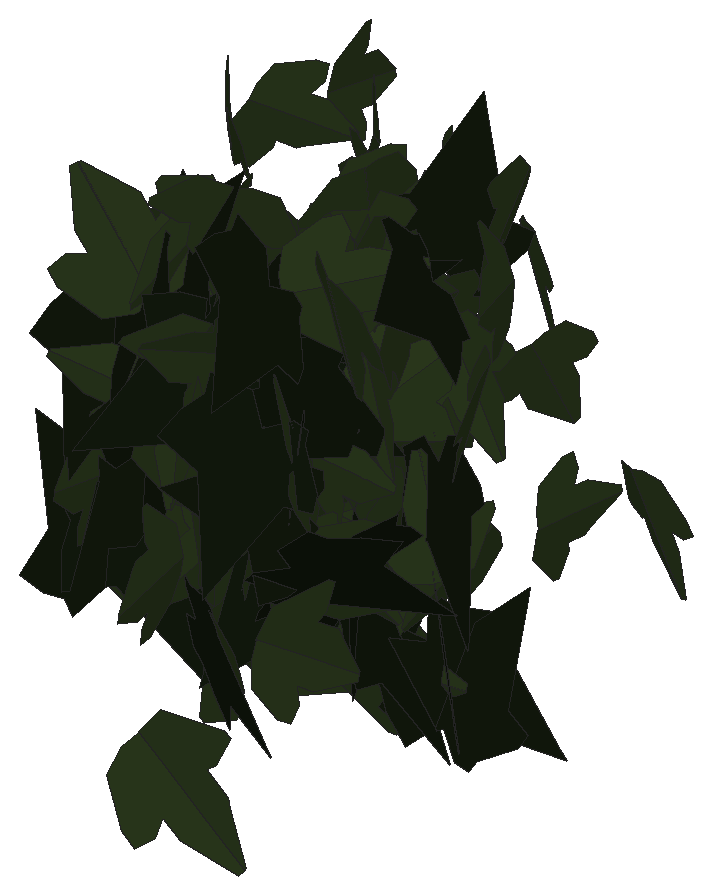
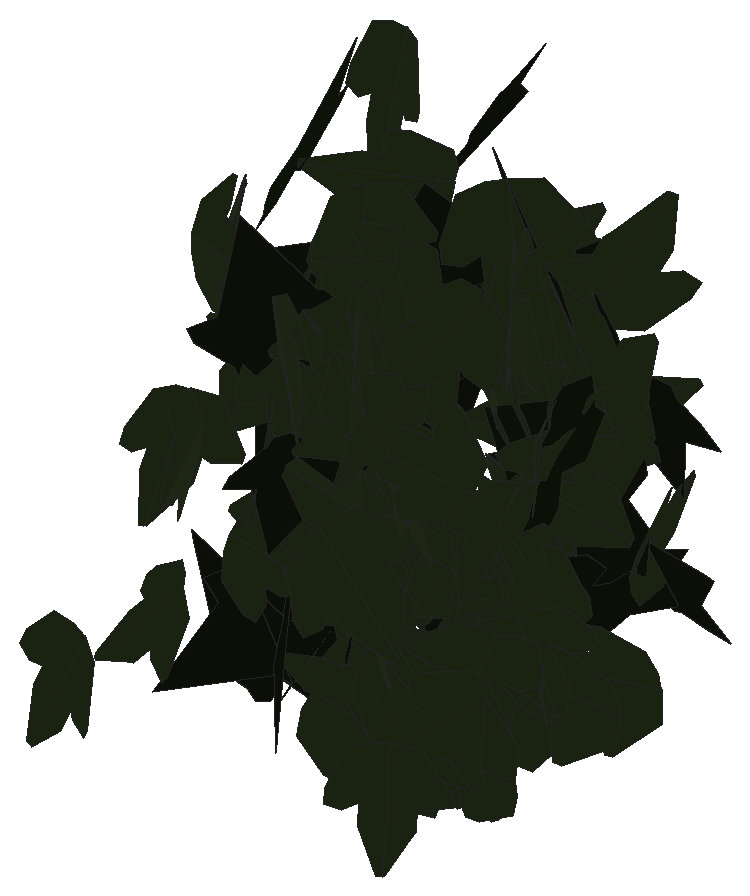
# SketchUp Ruby script. Lengths in inches.
U = 1.inch
M = Sketchup.active_model
def pt(a) = Geom::Point3d.new(a.map { |v| v * U })
def face(e, loops, mat)
  f = e.add_face(loops[0].map { |a| pt(a) })
  loops[1..].each { |l| e.add_face(l.map { |a| pt(a) }).erase! }
  f.material = f.back_material = mat if mat
  f
end
# faces: each face lists its corners as indices into pts; further lists are holes
def faces(e, pts, list, mat = nil) = list.each { |f| face(e, (f[0].is_a?(Array) ? f : [f]).map { |l| l.map { |i| pts[i] } }, mat) }
# xy, xz, yz: faces in a plane at the given z, y or x. An outline is a flat list of corners, or four numbers for a rectangle; further outlines are holes
def ring(l) = l.size == 4 ? [[l[0], l[1]], [l[2], l[1]], [l[2], l[3]], [l[0], l[3]]] : l.each_slice(2).to_a
def flat(e, list, mat, &to3) = list.each { |f| face(e, (f[0].is_a?(Array) ? f : [f]).map { |l| ring(l).map { |u, v| to3.(u, v) } }, mat) }
def xy(e, z, list, mat = nil) = flat(e, list, mat) { |x, y| [x, y, z] }
def xz(e, y, list, mat = nil) = flat(e, list, mat) { |x, z| [x, y, z] }
def yz(e, x, list, mat = nil) = flat(e, list, mat) { |y, z| [x, y, z] }
def lines(e, pts, list) = list.each { |a, b| e.add_line(pt(pts[a]), pt(pts[b])) }
# prism: a flat outline (further loops are holes) pulled along v
def prism(e, loops, v, mat = nil)
  f = face(e, loops, mat); d = Geom::Vector3d.new(v.map { |x| x * U })
  f.pushpull(f.normal.samedirection?(d) ? d.length : -d.length)
end
def box(e, o, s, mat = nil) = prism(e, [[o, [o[0] + s[0], o[1], o[2]], [o[0] + s[0], o[1] + s[1], o[2]], [o[0], o[1] + s[1], o[2]]]], [0, 0, s[2]], mat)
def at(x, y, z, deg = 0) = Geom::Transformation.translation(pt([x, y, z])) * Geom::Transformation.rotation(ORIGIN, Z_AXIS, deg.degrees)
def axes(o, x, y, z) = Geom::Transformation.new([*x, 0, *y, 0, *z, 0, *pt(o).to_a, 1])
def part(name) = M.definitions.add(name)
# library, detail: a bought-in or finely detailed component or shape, given as its bounding box
def library(name, o, s) = part(name).tap { |d| box(d.entities, o, s) }
def detail(e, o, s) = box(e.add_group.entities, o, s)
def put(e, d, t, mat = nil) = e.add_instance(d, t).tap { |i| i.material = mat if mat }
def group(e, t, mat = nil) = e.add_group.tap { |g| g.transformation = t; g.material = mat if mat }.entities
root = M.entities
M.materials.add("efeu1").color = [18, 25, 13]
M.materials.add("efeu2").color = [43, 57, 29]
c1 = part("ivyleaf_10")
p = [[0,0.5,-0.03],[-0.0625,2.02,-0.43],[-0.19,2.01,-0.46],[-0.54,1.05,-0.29],[-0.52,0.625,-0.18],[-0.83,0.76,-0.28],
  [-1.16,0.64,-0.33],[-1.15,0.33,-0.24],[-0.77,-0.39,0.02],[-0.3,-0.51,0.16],[0.04,-0.48,0.23],[-0.02,2.01,-0.4375],
  [-0.06,2.01,-0.43],[0.04,-0.49,0.23],[0.67,-0.49,0.14],[1.38,0.36,-0.2],[1.375,0.51,-0.24],[0.81,0.65,-0.19],
  [0.62,0.59,-0.15],[0.6,1.09,-0.28],[0.5,1.23,-0.31]]
faces(c1.entities,p,[[0,1,2,3,4,5,6,7,8,9,10],[11,12,0,13,14,15,16,17,18,19,20]],"efeu2")
c2 = part("ivyleaf_9")
p = [[1.54,2.16,1.25],[1.36,2.04,1.19],[-0.21,0.99,0.68],[-0.71,1.11,0.82],[-0.85,0.86,0.67],[-0.8,0.17,0.21],
  [-0.9,-0.01,0.1],[-0.67,-0.16,-0.02],[-0.08,-0.08,-0.05],[-0.03,-0.6,-0.4],[0.65,-0.88,-0.66],[0.83,-0.6,-0.49],
  [1.29,-0.42,-0.43],[1.8125,-0.07,-0.26],[1.21,0.44,0.15]]
faces(c2.entities,p,[[0,1,2,3,4,5,6,7,8,9,10,11,12,13,14]],"efeu1")
put(root,c1,axes([519.99,138.27,161.49],[0.01708,0.59871,0.28931],[-0.01586,0.28969,-0.59856],[-0.66476,0.00847,0.02171]))
put(root,c2,axes([520.64,134.83,158.97],[-0.68317,0.00659,-0.40656],[-0.40655,0.0026,0.6832],[0.00699,0.79498,0.00113]))
put(root,c1,axes([519.92,136.04,161.66],[0.04006,-0.18559,-0.70803],[0.37652,0.61331,-0.13946],[0.62769,-0.35605,0.12884]))
put(root,c1,axes([520.33,137.07,161.02],[-0.19678,-0.41139,0.58645],[-0.08817,-0.58964,-0.44322],[0.71091,-0.187,0.10736]))
put(root,c1,axes([520.05,135.45,159.49],[-0.20688,0.19724,0.66334],[0.31587,-0.58911,0.27368],[0.61575,0.36846,0.08247]))
put(root,c1,axes([520.5,136.82,161.71],[-0.02052,0.28492,-0.66438],[-0.22356,0.62956,0.27689],[0.68746,0.21324,0.07022]))
put(root,c2,axes([520.31,135.49,161.83],[-0.65787,-0.20013,-0.33798],[0.3227,0.10049,-0.68763],[0.22393,-0.73275,-0.002]))
put(root,c1,axes([519.74,136.18,158.18],[-0.0427,-0.04966,-0.72084],[0.72221,-0.0251,-0.04105],[-0.02218,-0.72167,0.05103]))
put(root,c1,axes([519.98,136.39,162.16],[-0.60774,-0.06485,0.47413],[0.47185,0.04655,0.61119],[-0.07978,0.76941,0.00299]))
put(root,c1,axes([520.47,139.94,163.27],[-0.029,0.13804,0.62277],[-0.22864,0.57975,-0.13915],[-0.59551,-0.22931,0.02309]))
put(root,c1,axes([520.49,139.93,158.375],[-0.59029,-0.23675,0.0375],[-0.03446,-0.01482,-0.63599],[0.23721,-0.59129,0.00093]))
put(root,c1,axes([520.64,137.43,164.05],[-0.39656,0.33601,0.42889],[-0.36509,0.22987,-0.51767],[-0.40442,-0.537,0.04677]))
put(root,c1,axes([520.41,137.34,159.18],[0.53822,0.37125,-0.16576],[-0.13837,-0.09132,-0.65384],[-0.38231,0.55572,0.00329]))
put(root,c1,axes([519.87,136.8125,158.13],[0.11344,-0.10818,-0.72291],[0.72947,-0.02992,0.11895],[-0.04664,-0.73114,0.1021]))
put(root,c1,axes([520.35,138.125,159.29],[0.4666,0.42819,0.2143],[0.15386,0.14928,-0.63327],[-0.45343,0.49128,0.00564]))
put(root,c1,axes([520.09,138.34,157.8],[0.0085,-0.05379,0.66221],[0.63696,0.18898,0.00718],[-0.18893,0.63473,0.05398]))
put(root,c1,axes([520.78,135.31,162.74],[0.38275,0.68648,0.29535],[-0.15889,-0.24949,0.7858],[0.73023,-0.4141,0.01618]))
put(root,c1,axes([520.94,136.16,161.14],[-0.15496,0.1411,0.62925],[-0.45745,0.43209,-0.20955],[-0.45453,-0.48298,-0.00364]))
put(root,c1,axes([520.97,135.35,161.01],[0.21123,0.25243,0.6061],[-0.39918,-0.45613,0.32909],[0.52128,-0.45158,0.0064]))
put(root,c2,axes([520.09,137.1,161.4375],[0.32452,-0.47834,0.56114],[0.34006,-0.4469,-0.57761],[0.65425,0.46954,0.02189]))
put(root,c1,axes([520.23,137.06,159.72],[0.19932,0.20882,0.65979],[0.47349,0.4596,-0.28851],[-0.50471,0.51364,-0.01009]))
put(root,c1,axes([521,136.41,158.51],[0.00537,-0.03455,-0.71906],[-0.34732,0.62973,-0.03285],[0.63056,0.34716,-0.01197]))
put(root,c1,axes([520.47,136.54,161.07],[-0.35145,-0.24689,-0.47886],[0.39212,0.27487,-0.4295],[0.36947,-0.52657,0.00032]))
put(root,c1,axes([520.43,138.42,158.55],[-0.22462,-0.15234,-0.61295],[0.50576,0.34629,-0.2714],[0.37832,-0.5534,-0.0011]))
put(root,c2,axes([520.7,135.62,162.89],[-0.55215,0.07007,-0.54246],[0.53765,-0.07208,-0.55658],[-0.10049,-0.77067,0.00273]))
put(root,c1,axes([520.57,138.27,163.84],[-0.2446,-0.28556,-0.55332],[0.39403,0.38932,-0.37511],[0.48213,-0.46305,0.02585]))
put(root,c2,axes([520.59,135.59,159.16],[-0.05391,-0.64343,-0.47983],[0.09533,0.47238,-0.64414],[0.79696,-0.10003,0.0446]))
put(root,c1,axes([520.75,136.93,159.86],[-0.12088,-0.15799,-0.70736],[0.44006,0.55382,-0.19889],[0.5759,-0.45634,0.00351]))
put(root,c2,axes([520.42,135.47,160.2],[0.33125,0.01219,-0.69677],[0.63915,0.30213,0.30914],[0.27772,-0.70988,0.11961]))
put(root,c1,axes([521.37,138.15,158.2],[-0.54105,-0.15447,0.32085],[-0.29273,-0.13937,-0.56073],[0.20276,-0.61339,0.04661]))
put(root,c1,axes([521.08,136.29,163.16],[-0.06743,-0.24557,0.71648],[0.15241,-0.709,-0.22866],[0.7419,0.12334,0.11209]))
put(root,c1,axes([521.21,137.15,160.24],[0.00049,-0.50295,-0.54014],[-0.00598,0.54012,-0.50294],[0.73802,0.00471,-0.00372]))
put(root,c1,axes([520.67,137.8,157.34],[0.07064,-0.00515,0.66044],[0.62376,-0.21782,-0.06842],[0.21711,0.62748,-0.01832]))
put(root,c1,axes([520.94,136.79,162.66],[0.04051,-0.51554,-0.51147],[0.13701,-0.49764,0.51245],[-0.71317,-0.12488,0.0694]))
put(root,c1,axes([520.82,138.35,161.56],[-0.19577,-0.21843,0.58171],[0.41634,0.40663,0.29281],[-0.46125,0.45975,0.0174]))
put(root,c1,axes([521.24,136.52,157.19],[-0.69559,0.17322,0.04012],[0.03859,-0.01106,0.71683],[0.17357,0.69665,0.00141]))
put(root,c1,axes([521.1,137.52,158.7],[0.09591,0.28812,-0.61732],[0.19522,0.58564,0.30366],[0.65267,-0.21751,-0.00011]))
put(root,c1,axes([521.82,138.27,158.5625],[-0.29793,-0.02674,0.67681],[-0.67077,-0.091,-0.29887],[0.09404,-0.73386,0.0124]))
put(root,c1,axes([520.83,137.5,160.125],[0.30535,-0.27764,-0.64369],[0.5492,-0.3416,0.40786],[-0.43566,-0.62521,0.06301]))
put(root,c1,axes([521.79,137.92,160.71],[0.28943,-0.04814,-0.61462],[-0.601,0.12923,-0.29315],[0.13735,0.66695,0.01244]))
put(root,c2,axes([521.09,135.82,162.58],[-0.20578,0.4459,0.58644],[0.24921,-0.53086,0.49109],[0.69328,0.32318,-0.00246]))
put(root,c1,axes([521.82,138.01,157.3],[-0.00114,0.06306,0.64759],[-0.55875,-0.33192,0.03134],[0.33339,-0.55607,0.05473]))
put(root,c1,axes([521.7,135.75,159.24],[0.49605,0.16839,0.49544],[-0.47092,-0.15398,0.52384],[0.22814,-0.68397,0.00404]))
put(root,c1,axes([521.69,138.92,163.51],[0.14697,-0.37067,-0.54822],[-0.17194,0.5209,-0.3983],[0.63905,0.2254,0.01892]))
put(root,c1,axes([521.55,136.13,158.79],[-0.10627,-0.15516,0.71497],[0.09974,-0.7188,-0.14117],[0.72479,0.07617,0.12425]))
put(root,c1,axes([521.6,136.2,161.3125],[0.66165,-0.25225,0.22653],[-0.20665,0.09376,0.70798],[-0.26878,-0.69304,0.01333]))
put(root,c1,axes([521.84,135.91,163.84],[-0.64415,-0.35748,0.14599],[-0.11827,-0.08764,-0.73645],[0.36758,-0.65465,0.01888]))
put(root,c1,axes([522.14,135.4,157.35],[-0.11537,0.08073,-0.70751],[-0.56188,0.43,0.14069],[0.43747,0.57357,-0.00589]))
put(root,c1,axes([521.67,138.08,161.36],[0.20897,-0.63713,0.11459],[0.0486,-0.10464,-0.6704],[0.64553,0.21413,0.01338]))
put(root,c1,axes([521.65,136.21,161.02],[0.50894,-0.53914,0.06018],[0.04759,-0.03784,-0.74136],[0.5404,0.51109,0.0086]))
put(root,c1,axes([521.76,136.36,158.83],[0.49435,-0.48104,-0.05138],[-0.03477,0.03795,-0.68976],[0.48252,0.49557,0.00294]))
put(root,c1,axes([521.68,136.16,162.07],[-0.06741,-0.53735,-0.38146],[0.06448,-0.38699,0.53375],[-0.65582,0.01718,0.09169]))
put(root,c1,axes([521.97,137.12,160.66],[-0.29654,0.42219,0.45509],[-0.25436,0.37743,-0.51589],[-0.56626,-0.39063,-0.00659]))
put(root,c1,axes([521.64,134.8,158.96],[-0.06862,0.04752,0.72748],[0.34451,-0.64185,0.07442],[0.6425,0.34924,0.03779]))
put(root,c1,axes([522.3,138.19,163.1],[0.14033,-0.14811,-0.68645],[-0.46084,0.50878,-0.20399],[0.52988,0.48171,0.00439]))
put(root,c1,axes([522.13,138.83,160.27],[-0.28128,-0.61616,0.34771],[-0.14735,-0.31495,-0.67732],[0.69198,-0.31753,-0.00289]))
put(root,c1,axes([522.12,134.85,162.42],[-0.26016,-0.54745,0.34009],[-0.14358,-0.30831,-0.60612],[0.62829,-0.29714,0.00231]))
put(root,c1,axes([521.36,135.76,159.32],[0.08009,-0.14421,-0.82456],[0.64085,-0.52234,0.1536],[-0.53853,-0.64302,0.06016]))
put(root,c1,axes([521.9,138.41,161.95],[0.42123,0.48824,-0.30348],[0.16492,0.25778,0.64363],[0.55071,-0.45065,0.03938]))
put(root,c1,axes([521.53,135.02,160.77],[-0.18914,-0.04208,-0.70449],[0.68997,0.14236,-0.19375],[0.14842,-0.71542,0.00288]))
put(root,c2,axes([522.1,137.03,158.34],[-0.3114,-0.63437,0.37839],[-0.16979,-0.33817,-0.70667],[0.71887,-0.35467,-0.003]))
put(root,c1,axes([521.98,137.32,162.4],[-0.06948,-0.44392,-0.63667],[0.23495,0.5972,-0.44204],[0.73974,-0.23137,0.0806]))
put(root,c2,axes([522.33,135.1875,161.95],[-0.40582,-0.44111,0.56041],[-0.37418,-0.41723,-0.59936],[0.60715,-0.55197,0.00519]))
put(root,c1,axes([522.5,137.08,159.05],[0.39563,-0.12717,-0.55307],[-0.53158,0.153,-0.41544],[0.19869,0.66257,-0.01022]))
put(root,c1,axes([522.01,134.57,161.68],[0.64181,-0.19109,0.18532],[0.17711,-0.05457,-0.66965],[0.19873,0.66579,-0.0017]))
put(root,c1,axes([522.02,137.97,158.34],[0.19449,-0.35192,-0.5134],[0.26258,-0.44129,0.40196],[-0.56434,-0.32661,0.01009]))
put(root,c1,axes([522.58,134.98,162.32],[-0.20365,-0.1579,-0.65503],[-0.36322,-0.55063,0.24566],[-0.56751,0.40908,0.07783]))
put(root,c1,axes([522.23,136.77,157.19],[0.25036,0.24696,-0.67012],[0.2806,0.61898,0.33294],[0.65674,-0.35861,0.1132]))
put(root,c2,axes([522.48,134.48,158.56],[0.60369,-0.26922,-0.47629],[-0.43618,0.19133,-0.66099],[0.33028,0.74477,-0.00236]))
put(root,c1,axes([522.32,137.81,163.26],[-0.16028,-0.17347,-0.66224],[0.44246,0.49276,-0.23616],[0.52239,-0.47058,-0.00316]))
put(root,c1,axes([522.79,139.03,163.31],[0.26348,-0.57507,-0.26481],[-0.11718,0.23757,-0.63252],[0.62217,0.28827,-0.00699]))
put(root,c1,axes([523.07,137.65,157.32],[-0.23182,-0.23583,0.59657],[-0.4,-0.44277,-0.33047],[0.50151,-0.46216,0.01219]))
put(root,c1,axes([522.69,137.98,162.21],[0.20131,-0.56917,0.33111],[-0.11746,0.30965,0.60369],[-0.64792,-0.23298,-0.00656]))
put(root,c1,axes([522.93,136.17,160.15],[0.02514,-0.42239,-0.48291],[0.03832,0.4834,-0.42083],[0.64043,-0.01235,0.04414]))
put(root,c1,axes([522.77,137.05,163.36],[-0.40143,-0.45576,-0.39586],[0.31348,0.24889,-0.60444],[0.5159,-0.50587,0.05926]))
put(root,c1,axes([522.97,137.21,163.99],[-0.2701,-0.61457,-0.11926],[0.05169,0.10755,-0.6713],[0.6239,-0.27498,0.00399]))
put(root,c1,axes([522.98,137.7,160.16],[0.26404,-0.52097,0.56106],[-0.21826,0.51764,0.58337],[-0.73387,-0.34139,0.02836]))
put(root,c1,axes([522.92,136.1,163],[0.23876,-0.56585,0.25066],[0.08827,-0.23479,-0.61409],[0.61256,0.25439,-0.00921]))
put(root,c1,axes([522.9,136.07,159.61],[0.28702,-0.56409,0.40028],[0.21169,-0.34093,-0.63226],[0.65848,0.35548,0.02879]))
put(root,c1,axes([523.1,137.15,162.98],[-0.1992,0.53611,0.3744],[-0.15947,0.33975,-0.57133],[-0.63416,-0.25383,0.02606]))
put(root,c2,axes([522.8125,138.43,161.38],[-0.05939,-0.67875,-0.36334],[0.05106,0.36014,-0.68113],[0.76819,-0.07641,0.01718]))
put(root,c2,axes([523.34,135.29,160.28],[0.003,0.00331,0.81473],[0.00548,0.81472,-0.00333],[-0.81472,0.00549,0.00298]))
put(root,c2,axes([522.74,136.05,162.47],[0.17119,0.07478,0.74828],[0.71929,0.20761,-0.18531],[-0.21939,0.739,-0.02366]))
put(root,c1,axes([522.72,137.35,158.79],[0.01102,0.0114,0.70069],[0.68872,0.12931,-0.01293],[-0.12948,0.68875,-0.00917]))
put(root,c2,axes([523.16,134.94,162.02],[0.01002,-0.07622,-0.85856],[-0.14769,0.84576,-0.07681],[0.84918,0.148,-0.00323]))
put(root,c2,axes([523.375,138.3125,162.51],[-0.54265,-0.20914,0.51751],[0.5173,0.08264,0.57584],[-0.20964,0.74529,0.08137]))
put(root,c1,axes([523.53,135.26,160.68],[-0.59779,0.61678,0.09343],[0.05908,-0.07284,0.8589],[0.62101,0.60065,0.00823]))
put(root,c1,axes([523.41,137.09,163.26],[0.02692,0.51211,-0.45605],[-0.04973,-0.45374,-0.51245],[-0.68393,0.05315,0.01931]))
put(root,c1,axes([523.58,137.91,162.21],[-0.27687,-0.64426,-0.03739],[0.02044,0.03191,-0.7012],[0.64502,-0.27755,0.00617]))
put(root,c2,axes([523.41,134.5,161.68],[-0.22758,-0.74793,0.15072],[-0.04768,-0.14304,-0.78178],[0.76148,-0.23249,-0.0039]))
put(root,c1,axes([523.22,136.11,159.3],[-0.44052,0.06542,-0.49262],[0.48981,-0.054,-0.44517],[-0.08392,-0.65865,-0.01243]))
put(root,c2,axes([523.1875,136.94,158.6875],[0.1469,-0.07044,-0.76366],[0.66924,-0.36794,0.16268],[-0.37452,-0.68511,-0.00885]))
put(root,c1,axes([523.42,140.05,161.99],[-0.41711,0.48435,-0.28142],[0.18228,-0.21441,-0.6392],[-0.52968,-0.4552,0.00164]))
put(root,c2,axes([523.41,134.66,163.72],[-0.0536,-0.62249,0.51238],[-0.04151,-0.5107,-0.62479],[0.80517,-0.06777,0.00189]))
put(root,c1,axes([523.78,138.03,160.54],[-0.17086,0.64674,-0.35605],[-0.09301,0.3437,0.66893],[0.73239,0.19453,0.00188]))
put(root,c1,axes([523.64,137.3125,159.73],[0.46226,-0.51846,-0.03595],[-0.0252,0.0257,-0.69461],[0.51909,0.46294,-0.0017]))
put(root,c1,axes([523.14,136.14,160.5625],[-0.02406,-0.06446,-0.64016],[0.6024,-0.22727,0.00025],[-0.22599,-0.59894,0.06881]))
put(root,c2,axes([523.81,134.84,160.52],[0.04809,-0.68008,-0.3633],[0.0572,-0.35985,0.6812],[-0.76891,-0.06931,0.02795]))
put(root,c1,axes([523.46,137.4,159.55],[-0.54499,-0.17404,0.38096],[0.36836,0.09836,0.5719],[-0.19933,0.65762,0.01528]))
put(root,c1,axes([523.34,136.77,161.46],[0.45236,-0.12723,0.46148],[0.45187,-0.09607,-0.46943],[0.15799,0.63904,0.02131]))
put(root,c1,axes([523.47,137.04,161.18],[0.37873,0.16976,-0.59681],[0.46814,0.38073,0.40538],[0.40724,-0.59554,0.08903]))
put(root,c1,axes([523.62,136.99,159.53],[-0.04927,-0.05383,0.68033],[0.35381,-0.58529,-0.02069],[0.58358,0.35031,0.06998]))
put(root,c1,axes([523.25,136.86,157.38],[-0.01374,0.02185,-0.77796],[0.76471,-0.14422,-0.01756],[-0.14464,-0.7646,-0.01892]))
put(root,c2,axes([523.625,136.52,158.32],[0.45992,-0.56043,-0.25866],[-0.15443,0.20783,-0.7249],[0.59761,0.48502,0.01174]))
put(root,c1,axes([523.97,136.62,162.76],[0.08242,-0.2596,-0.77329],[0.04351,0.77752,-0.25638],[0.81454,-0.01526,0.09194]))
put(root,c2,axes([524.15,135.08,159.83],[0.04803,0.80891,-0.11699],[-0.00716,-0.11677,-0.81033],[-0.81729,0.04856,0.00023]))
put(root,c1,axes([523.52,135.44,163.47],[0.16203,-0.02507,-0.72057],[0.64109,0.34296,0.13223],[0.32993,-0.6541,0.09695]))
put(root,c1,axes([524.08,134.77,159.79],[-0.26217,-0.36271,-0.63131],[0.37106,0.51075,-0.44754],[0.62644,-0.45433,0.00089]))
put(root,c1,axes([524.41,137.6,159.06],[-0.02902,-0.42579,0.51823],[-0.02002,-0.51794,-0.42667],[0.67042,-0.0339,0.0097]))
put(root,c1,axes([524.4375,136.86,159.29],[0.227,0.6509,0.02879],[-0.00959,-0.02714,0.68935],[0.65147,-0.22721,0.00011]))
put(root,c1,axes([524.01,137.71,161.71],[0.57463,0.06195,0.46136],[0.45409,0.08666,-0.57722],[-0.10242,0.73181,0.02929]))
put(root,c2,axes([524.74,136.58,158.2],[0.23329,0.0027,-0.75716],[-0.733,0.19936,-0.22514],[0.18975,0.76679,0.0612]))
put(root,c1,axes([524.3,138.6,163.74],[0.1789,-0.39575,0.50296],[0.24021,-0.44254,-0.43365],[0.5932,0.29856,0.02392]))
put(root,c1,axes([524.54,138.78,161.33],[-0.3112,-0.52985,-0.27677],[0.14322,0.23685,-0.61448],[0.58037,-0.34256,0.00323]))
put(root,c1,axes([524.56,139.01,158.86],[0.00876,-0.10271,-0.66128],[0.16214,0.64196,-0.09756],[0.64927,-0.15893,0.03328]))
put(root,c1,axes([524.83,134.36,164.2],[-0.70049,0.37854,0.14958],[-0.13193,0.07051,-0.79623],[-0.38505,-0.71281,0.00068]))
put(root,c2,axes([524.41,134.0625,160.27],[0.66517,0.38495,0.3228],[0.26716,0.18255,-0.76821],[-0.42546,0.71647,0.02229]))
put(root,c2,axes([524.33,136.875,157.86],[0.02014,-0.20481,-0.73651],[0.35965,0.65268,-0.17166],[0.67457,-0.34186,0.11351]))
put(root,c2,axes([524.61,136.8125,156.9],[-0.45014,0.16075,0.59626],[0.55109,-0.22842,0.47762],[0.2787,0.71132,0.01862]))
put(root,c2,axes([524.51,136.8,160.54],[-0.34574,-0.04026,-0.71456],[0.70765,0.0994,-0.348],[0.10699,-0.78756,-0.00739]))
put(root,c1,axes([524.28,131.33,158.6],[0.5026,0.17501,0.67755],[0.64269,0.21461,-0.53218],[-0.27687,0.81586,-0.00536]))
put(root,c1,axes([524.88,133.11,159.68],[0.02734,0.38404,0.64329],[-0.03329,0.6437,-0.38287],[-0.74846,-0.0146,0.04052]))
put(root,c1,axes([524.87,140.56,158.68],[-0.60546,0.31636,-0.20066],[0.17332,-0.10155,-0.68307],[-0.33213,-0.62971,0.00934]))
put(root,c1,axes([525.0625,136.88,161.93],[0.36427,-0.60825,0.00946],[0.00484,-0.00812,-0.70898],[0.6083,0.3643,-0.00002]))
put(root,c2,axes([524.79,136.26,163.6],[0.43543,-0.43084,-0.46948],[0.33787,-0.32601,0.61253],[-0.54026,-0.55112,0.00468]))
put(root,c1,axes([524.84,137.65,162.91],[-0.21013,0.10814,0.66432],[0.42454,-0.51874,0.21873],[0.52228,0.46517,0.08948]))
